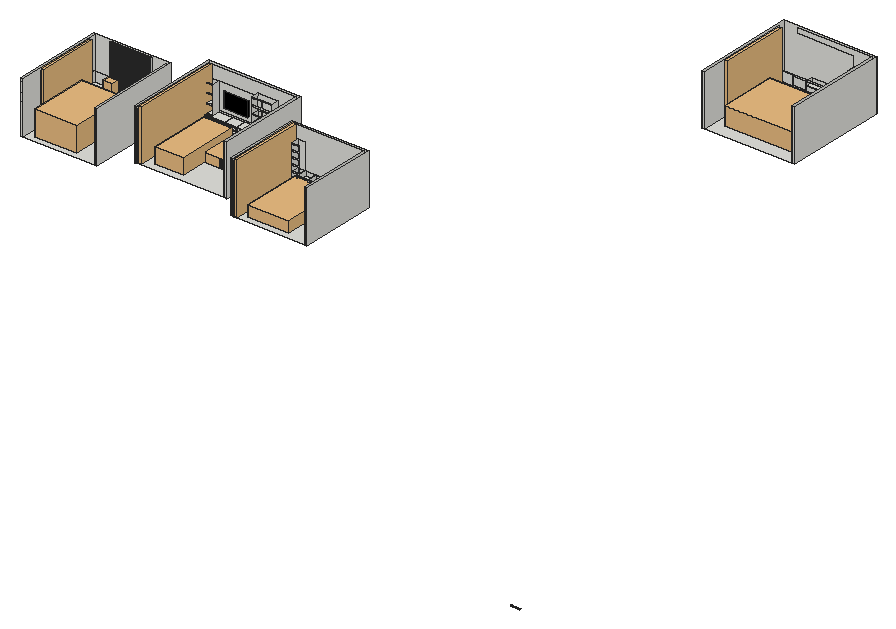
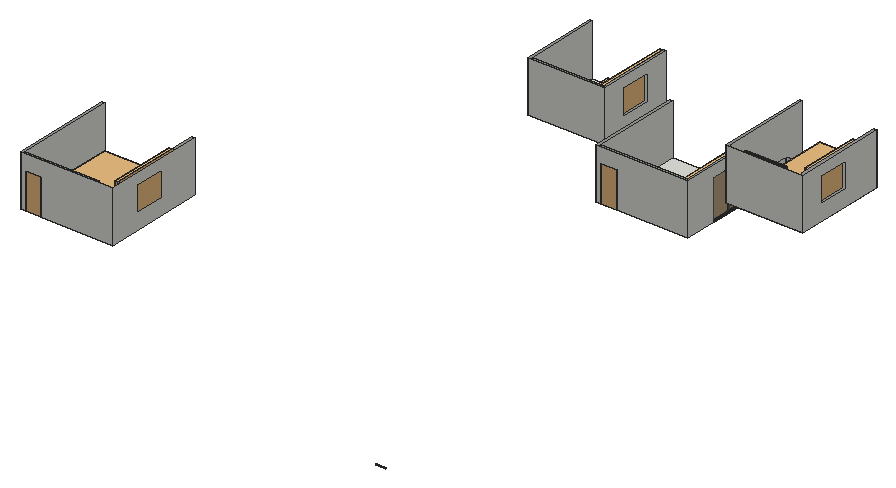
# SketchUp Ruby script. Lengths in inches.
U = 1.inch
M = Sketchup.active_model
def pt(a) = Geom::Point3d.new(a.map { |v| v * U })
def face(e, loops, mat)
  f = e.add_face(loops[0].map { |a| pt(a) })
  loops[1..].each { |l| e.add_face(l.map { |a| pt(a) }).erase! }
  f.material = f.back_material = mat if mat
  f
end
# faces: each face lists its corners as indices into pts; further lists are holes
def faces(e, pts, list, mat = nil) = list.each { |f| face(e, (f[0].is_a?(Array) ? f : [f]).map { |l| l.map { |i| pts[i] } }, mat) }
# xy, xz, yz: faces in a plane at the given z, y or x. An outline is a flat list of corners, or four numbers for a rectangle; further outlines are holes
def ring(l) = l.size == 4 ? [[l[0], l[1]], [l[2], l[1]], [l[2], l[3]], [l[0], l[3]]] : l.each_slice(2).to_a
def flat(e, list, mat, &to3) = list.each { |f| face(e, (f[0].is_a?(Array) ? f : [f]).map { |l| ring(l).map { |u, v| to3.(u, v) } }, mat) }
def xy(e, z, list, mat = nil) = flat(e, list, mat) { |x, y| [x, y, z] }
def xz(e, y, list, mat = nil) = flat(e, list, mat) { |x, z| [x, y, z] }
def yz(e, x, list, mat = nil) = flat(e, list, mat) { |y, z| [x, y, z] }
def lines(e, pts, list) = list.each { |a, b| e.add_line(pt(pts[a]), pt(pts[b])) }
# prism: a flat outline (further loops are holes) pulled along v
def prism(e, loops, v, mat = nil)
  f = face(e, loops, mat); d = Geom::Vector3d.new(v.map { |x| x * U })
  f.pushpull(f.normal.samedirection?(d) ? d.length : -d.length)
end
def box(e, o, s, mat = nil) = prism(e, [[o, [o[0] + s[0], o[1], o[2]], [o[0] + s[0], o[1] + s[1], o[2]], [o[0], o[1] + s[1], o[2]]]], [0, 0, s[2]], mat)
def at(x, y, z, deg = 0) = Geom::Transformation.translation(pt([x, y, z])) * Geom::Transformation.rotation(ORIGIN, Z_AXIS, deg.degrees)
def axes(o, x, y, z) = Geom::Transformation.new([*x, 0, *y, 0, *z, 0, *pt(o).to_a, 1])
def part(name) = M.definitions.add(name)
# library, detail: a bought-in or finely detailed component or shape, given as its bounding box
def library(name, o, s) = part(name).tap { |d| box(d.entities, o, s) }
def detail(e, o, s) = box(e.add_group.entities, o, s)
def put(e, d, t, mat = nil) = e.add_instance(d, t).tap { |i| i.material = mat if mat }
def group(e, t, mat = nil) = e.add_group.tap { |g| g.transformation = t; g.material = mat if mat }.entities
root = M.entities
M.materials.add("Chrome_Polished").color = [2, 2, 2]
M.materials.add("[0135_DarkGray]").color = [81, 81, 81]
M.materials.add("[0137_Black]").color = [0, 0, 0]
M.materials.add("[Translucent Glass Gray]").color = [128, 128, 128]
M.materials["[Translucent Glass Gray]"].alpha = 0.15
M.materials.add("blackened steel1").color = [30, 30, 30]
c1 = part("Horizontal batten")
box(c1.entities,[0,-1,0],[23,1,1])
c2 = library("Garniza_zaclona",[1.52,0,0],[127.96,8.15,78.72])
c3 = library("main+door",[0,-0.79,0],[47.24,7.88,82.68])
c4 = part("PENTEK_RP Fineline 50S_SlidingDoor_Glass")
box(c4.entities,[0,0,0],[46.58,0.16,94.39],"[Translucent Glass Gray]")
c5 = part("PENTEK_RP Fineline 50S_SlidingDoor_GlazingBead")
box(c5.entities,[0,0,0],[45.47,0.59,0.56],"[0135_DarkGray]")
c6 = part("PENTEK_RP Fineline 50S_SlidingDoor_GlazingBead_2")
box(c6.entities,[0,0,0],[0.56,0.59,94.39],"[0135_DarkGray]")
c7 = part("PENTEK_RP Fineline 50S_SlidingDoor_Leaf_E1")
xy(c7.entities,0,[[0,0,0.93,1.97],[0.93,1.57,1.49,1.97]],"[0135_DarkGray]")
xy(c7.entities,96.25,[[0,0,0.93,0,0.93,1.57,1.49,1.57,1.49,1.97,0,1.97]],"[0135_DarkGray]")
xz(c7.entities,0,[[0,0,0.93,96.25]],"[0135_DarkGray]")
xz(c7.entities,1.57,[[0.93,0,1.49,95.32],[0.93,95.32,1.49,96.25]],"[0135_DarkGray]")
xz(c7.entities,1.97,[[0,0,1.49,96.25]],"[0135_DarkGray]")
yz(c7.entities,0,[[0,0,1.97,96.25]],"[0135_DarkGray]")
yz(c7.entities,0.93,[[0,0,1.57,0.93],[0,0.93,1.57,95.32],[0,95.32,1.57,96.25]],"[0135_DarkGray]")
yz(c7.entities,1.49,[[1.57,0,1.97,95.32],[1.57,95.32,1.97,96.25]],"[0135_DarkGray]")
c8 = part("PENTEK_RP Fineline 50S_SlidingDoor_Leaf_E2")
xy(c8.entities,0,[[0,0,0,1.57,0.56,1.57,0.56,1.97,46.02,1.97,46.02,1.57,46.58,1.57,46.58,0]],"[0135_DarkGray]")
xy(c8.entities,0.93,[[0,0,46.58,1.57]],"[0135_DarkGray]")
xy(c8.entities,1.49,[[0.56,1.57,46.02,1.97]],"[0135_DarkGray]")
xz(c8.entities,0,[[0,0,46.58,0.93]],"[0135_DarkGray]")
xz(c8.entities,1.57,[[0,0,0.56,0.93],[46.02,0,46.58,0.93],[0.56,0.93,46.02,1.49]],"[0135_DarkGray]")
xz(c8.entities,1.97,[[0.56,0,46.02,1.49]],"[0135_DarkGray]")
yz(c8.entities,0,[[0,0,1.57,0.93]],"[0135_DarkGray]")
yz(c8.entities,0.56,[[1.57,0,1.97,0.93],[1.57,0.93,1.97,1.49]],"[0135_DarkGray]")
yz(c8.entities,46.02,[[1.57,0,1.97,0.93],[1.57,0.93,1.97,1.49]],"[0135_DarkGray]")
yz(c8.entities,46.58,[[0,0,1.57,0.93]],"[0135_DarkGray]")
c9 = part("PENTEK_RP Fineline 50S_SlidingDoor_Leaf2")
put(c9.entities,c4,at(1.49,1.42,0.93))
put(c9.entities,c5,at(1.49,0,94.77))
put(c9.entities,c6,at(46.96,0,0.93))
put(c9.entities,c4,at(1.49,0.59,0.93))
put(c9.entities,c6,at(0.93,0,0.93))
put(c9.entities,c7,at(0,0,0))
put(c9.entities,c7,axes([48.44,0,0],[-1,0,0],[0,1,0],[0,0,1]))
put(c9.entities,c5,at(1.49,0,0.93))
put(c9.entities,c8,axes([0.93,0,96.25],[1,0,0],[0,1,0],[0,0,-1]))
put(c9.entities,c8,at(0.93,0,0))
c10 = part("PENTEK_RP Fineline S_SlidingDoor_Leaf1")
put(c10.entities,c6,at(0.93,0,0.93))
put(c10.entities,c6,at(46.96,0,0.93))
put(c10.entities,c4,at(1.49,1.42,0.93))
put(c10.entities,c5,at(1.49,0,0.93))
put(c10.entities,c4,at(1.49,0.59,0.93))
put(c10.entities,c7,at(0,0,0))
put(c10.entities,c7,axes([48.44,0,0],[-1,0,0],[0,1,0],[0,0,1]))
put(c10.entities,c8,axes([0.93,0,96.25],[1,0,0],[0,1,0],[0,0,-1]))
put(c10.entities,c8,at(0.93,0,0))
put(c10.entities,c5,at(1.49,0,94.77))
c11 = part("PENTEK_RP Fineline 50S_Sliding_DoorCase_E1")
box(c11.entities,[0,0,0],[1.51,3.66,99.27],"[0135_DarkGray]")
c12 = part("PENTEK_RP Fineline 50S_SlidingDooe_Case_E2")
box(c12.entities,[0,0,0],[96.25,3.66,1.51],"[0135_DarkGray]")
c13 = part("pentek_RP Fineline 50S_SlidingDoor_Case")
put(c13.entities,c11,at(97.76,0,0))
put(c13.entities,c12,at(1.51,0,0))
put(c13.entities,c11,at(0,0,0))
put(c13.entities,c12,at(1.51,0,97.76))
c14 = library("2222",[-1.18,-2.36,0.79],[68.11,146.45,37.25])
c15 = library("Group\#8",[0,0,0],[54,72,22])
c16 = part("Vertical batten")
box(c16.entities,[0,-1,0],[1,1,17])
c17 = part("Vertical batten \#1")
box(c17.entities,[-1,0,0],[1,1,16])
c18 = library("Garniza_zaclona\#1",[1.52,0,0],[127.96,8.15,78.72])
c19 = library("Garniza_zaclona\#3",[1.52,0,0],[127.96,8.15,78.72])
c20 = library("Garniza_zaclona\#2",[1.52,0,0],[127.96,8.15,78.72])
c21 = library("04+Sofa+y+Mesas",[-94.93,-111.67,3.93],[153.81,110.61,64.28])
c22 = library("Sofa+Set+3+(1)",[-143.38,0,-0.17],[159.32,111.7,30.39])
c23 = library("sofa+(2)",[-100.93,-81.02,-0.06],[174.43,145.32,46.54])
c24 = library("SKT_Nearly Natural 5' Kentia Palm Silk Tree",[-23.18,-17.61,0],[47.48,43.95,59.125])
c25 = part("Vertical wall batten")
prism(c25.entities,[[[1,0,0],[0,0,0],[0,0,24],[0,0,25],[0,0,48.5],[0,0,49.5],[0,0,73],[0,0,74],[0,0,98],[1,0,98]]],[0,-1,0])
xy(root,-33.45,[[194.45,99.3,398.45,99.3,398.45,309.3,392.45,309.3,392.45,315.3,356.45,315.3,356.45,309.3,194.45,309.3,194.45,243.3,188.45,243.3,188.45,147.3,194.45,147.3]])
xy(root,-28.45,[[194.45,285.3,218.45,309.3],[218.45,285.3,308.45,309.3],[308.45,285.3,332.45,309.3],[332.45,285.3,356.45,309.3]])
xy(root,-27.45,[[218.45,285.3,248.45,285.48],[249.45,285.3,277.45,309.3],[278.45,285.3,332.45,285.48]])
xy(root,-27.25,[[218.65,285.3,248.25,285.48],[278.65,285.3,308.25,285.48],[308.65,285.3,332.25,285.48]])
xy(root,-19.95,[[249.45,285.3,277.45,309.3]])
xy(root,-18.95,[[249.45,285.3,277.45,309.3]])
xy(root,-11.65,[[218.65,285.3,248.25,285.48],[278.65,285.3,308.25,285.48],[308.65,285.3,332.25,285.48]])
xy(root,-11.45,[[218.45,285.3,248.45,285.48],[249.45,285.3,277.45,309.3],[278.45,285.3,332.45,285.48]])
xy(root,-10.45,[[194.45,285.3,356.45,285.3,356.45,291.3,308.45,291.3,308.45,309.3,218.45,309.3,218.45,291.3,194.45,291.3]])
xy(root,-9.45,[[195.45,291.3,217.45,307.3],[309.45,291.3,355.45,309.3]])
xy(root,-4.45,[[218.45,307.3,308.45,309.3]])
xy(root,0,[[0.24,0,6.24,0,6.24,210,174.24,210,174.24,0,180.24,0,180.24,216,0.24,216],[6.24,0,174.24,210],[492.34,7.4375,660.34,7.4375,660.34,181.4375,522.34,181.4375,522.34,163.4375,504.34,163.4375,504.34,181.4375,492.34,181.4375],[962.01,801.86,1166.01,801.86,1166.01,1035.86,1160.01,1035.86,1160.01,1041.86,1124.01,1041.86,1124.01,1035.86,962.01,1035.86]])
xy(root,1,[[505.34,163.4375,521.34,181.4375]])
xy(root,4,[[6.24,192,174.24,210]])
xy(root,5,[[7.24,192,173.24,192.18]])
xy(root,5.2,[[7.4375,192,42.04,192.18],[42.4375,192,90.04,192.18],[90.4375,192,138.04,192.18],[138.4375,192,173.04,192.18]])
xy(root,6,[[156.24,48,174.24,156],[522.34,157.62,547.84,181.4375],[547.84,157.62,573.34,181.4375],[573.34,157.62,598.84,181.4375],[598.84,157.62,624.34,181.4375],
  [962.01,1017.86,1124.01,1035.86]])
xy(root,6.2,[[522.54,157.4375,547.64,157.62],[548.04,157.4375,573.34,157.62],[573.34,157.4375,598.64,157.62],[599.04,157.4375,624.14,157.62]])
xy(root,7,[[963.01,1017.86,1123.01,1018.04]])
xy(root,7.05,[[309.45,291.3,331.95,309.3],[331.95,291.3,332.95,309.3],[332.95,291.3,355.45,309.3]])
xy(root,7.2,[[963.21,1017.86,994.8125,1018.04],[995.21,1017.86,1026.8125,1018.04],[1027.21,1017.86,1058.8125,1018.04],[1059.21,1017.86,1090.8125,1018.04],[1091.21,1017.86,1122.8125,1018.04]])
xy(root,8,[[156.24,85.33,174.24,118.67]])
xy(root,8.05,[[309.45,291.3,331.95,309.3],[332.95,291.3,355.45,309.3]])
xy(root,11.05,[[195.45,291.3,217.45,307.3]])
xy(root,12.05,[[195.45,291.3,217.45,307.3]])
xy(root,14.5,[[156.24,85.33,174.24,118.67]])
xy(root,15.17,[[505.34,163.4375,521.34,181.4375]])
xy(root,15.5,[[156.24,85.33,174.24,118.67]])
xy(root,16.17,[[505.34,163.4375,521.34,181.4375]])
xy(root,17.8,[[522.54,157.4375,547.64,157.62],[548.04,157.4375,598.64,157.62],[599.04,157.4375,624.14,157.62],[1027.21,1017.86,1058.8125,1018.04],[1059.21,1017.86,1090.8125,1018.04]])
xy(root,18,[[522.34,157.4375,624.34,157.62],[1027.01,1017.86,1091.01,1018.04]])
xy(root,19,[[523.34,157.4375,547.34,181.4375],[548.34,157.4375,598.34,181.4375],[599.34,157.4375,623.34,181.4375],[1028.01,1017.86,1090.01,1033.86]])
xy(root,20.8,[[7.4375,192,42.04,192.18],[42.4375,192,90.04,192.18],[90.4375,192,138.04,192.18],[138.4375,192,173.04,192.18]])
xy(root,21,[[7.24,192,173.24,192.18]])
xy(root,22,[[156.24,85.33,174.24,118.67],[6.24,192,174.24,210]])
xz(root,0,[[0.24,0,6.24,120],[174.24,0,180.24,120]])
xz(root,7.4375,[[486.34,0,492.34,120],[660.34,0,666.34,120]])
xz(root,48,[[156.24,6,174.24,24]])
xz(root,85.33,[[156.24,8,174.24,14.5],[156.24,15.5,174.24,22]])
xz(root,99.3,[[188.45,-34.45,194.45,-33.45,194.45,85.55,188.45,85.55],[404.45,-34.45,404.45,85.55,398.45,85.55,398.45,-33.45]])
xz(root,118.67,[[156.24,8,174.24,14.5],[156.24,15.5,174.24,22]])
xz(root,147.3,[[188.45,-33.45,194.45,61.55]])
xz(root,156,[[156.24,6,174.24,24]])
xz(root,157.4375,[[522.54,6.2,547.64,17.8],[548.04,6.2,598.64,17.8],[599.04,6.2,624.14,17.8],[[522.34,18,624.34,30],[523.34,19,623.34,29]],[547.34,19,548.34,29],
  [598.34,19,599.34,29]])
xz(root,157.62,[[[522.34,6,624.34,18],[548.04,6.2,598.64,17.8],[599.04,6.2,624.14,17.8],[522.54,6.2,547.64,17.8]]])
xz(root,163.4375,[[[504.34,0,522.34,90],[505.34,1,521.34,15.17],[505.34,74.83,521.34,89],[505.34,16.17,521.34,29.83],[505.34,45.5,521.34,59.17],[505.34,30.83,521.34,44.5],[505.34,60.17,521.34,73.83]]])
xz(root,181.4375,[[492.34,0,504.34,0,504.34,90,523.34,90,523.34,30,624.34,30,624.34,6,522.34,6,522.34,0,660.34,0,660.34,120,492.34,120],[505.34,1,521.34,15.17],[505.34,16.17,521.34,29.83],[523.34,19,547.34,29],[548.34,19,598.34,29],
  [599.34,19,623.34,29]])
xz(root,187.4375,[[486.34,0,666.34,120]])
xz(root,192,[[[6.24,4,174.24,22],[7.24,5,173.24,21]],[7.4375,5.2,42.04,20.8],[42.4375,5.2,90.04,20.8],[90.4375,5.2,138.04,20.8],[138.4375,5.2,173.04,20.8]])
xz(root,192.18,[[[7.24,5,173.24,21],[90.4375,5.2,138.04,20.8],[42.4375,5.2,90.04,20.8],[138.4375,5.2,173.04,20.8],[7.4375,5.2,42.04,20.8]]],"Chrome_Polished")
xz(root,210,[[6.24,0,174.24,4],[6.24,22,42.24,46],[42.24,22,43.24,120],[43.24,22,138.24,120],[138.24,22,174.24,46]])
xz(root,216,[[0.24,0,180.24,120]])
xz(root,243.3,[[188.45,-33.45,194.45,61.55]])
xz(root,285.3,[[[194.45,-28.45,218.45,-28.45,218.45,-27.45,195.45,-27.45,195.45,-11.45,248.45,-11.45,248.45,-27.45,218.45,-27.45,218.45,-28.45,332.45,-28.45,332.45,-27.45,278.45,-27.45,278.45,-11.45,355.45,-11.45,355.45,-27.45,332.45,-27.45,332.45,-28.45,356.45,-28.45,356.45,-10.45,194.45,-10.45],[249.45,-27.45,277.45,-11.45]],[195.45,-27.45,218.45,-12.45],[332.45,-27.45,355.45,-11.45],[218.65,-27.25,248.25,-11.65],[278.65,-27.25,308.25,-11.65],
  [308.65,-27.25,332.25,-11.65],[249.45,-19.95,277.45,-18.95]])
xz(root,285.48,[[[218.45,-27.45,248.45,-11.45],[218.65,-27.25,248.25,-11.65]],[[278.45,-27.45,332.45,-11.45],[278.65,-27.25,308.25,-11.65],[308.65,-27.25,332.25,-11.65]]])
xz(root,291.3,[[[194.45,-10.45,218.45,55.55],[195.45,12.05,217.45,33.05],[195.45,-9.45,217.45,11.05],[195.45,34.05,217.45,54.55]],[[308.45,-10.45,356.45,61.55],[309.45,8.05,309.45,25.05,331.95,25.05,331.95,8.05,332.95,8.05,332.95,25.05,355.45,25.05,355.45,8.05],[309.45,-9.45,355.45,7.05],[332.95,26.05,355.45,43.05],[309.45,26.05,331.95,43.05],[309.45,44.05,331.95,60.55],[332.95,44.05,355.45,60.55]]])
xz(root,307.3,[[195.45,-9.45,217.45,11.05],[218.45,-4.45,308.45,55.55],[195.45,12.05,217.45,33.05]])
xz(root,309.3,[[194.45,-33.45,356.45,-28.45],[392.45,-33.45,398.45,-33.45,398.45,85.55,195.45,85.55,195.45,55.55,308.45,55.55,308.45,61.55,356.45,61.55,356.45,49.55,392.45,49.55],[249.45,-27.45,277.45,-19.95],[249.45,-18.95,277.45,-11.45],[218.45,-10.45,308.45,-4.45],
  [309.45,-9.45,355.45,7.05],[309.45,8.05,331.95,25.05],[332.95,8.05,355.45,25.05]])
xz(root,315.3,[[188.45,-34.45,188.45,85.55,404.45,85.55,404.45,-34.45,392.45,-33.45,392.45,49.55,356.45,49.55,356.45,-33.45]])
xz(root,801.86,[[956.01,0,962.01,120],[1166.01,0,1172.01,120]])
xz(root,1017.86,[[[962.01,6,1124.01,30],[963.01,7,1123.01,29]],[963.21,7.2,994.8125,28.8],[995.21,7.2,1026.8125,28.8],[1027.21,7.2,1058.8125,17.8],[1059.21,7.2,1090.8125,17.8],
  [1091.21,7.2,1122.8125,28.8],[[1027.01,18,1091.01,29],[1028.01,19,1090.01,28]]])
xz(root,1018.04,[[[963.01,7,1123.01,7,1123.01,29,1091.01,29,1091.01,18,1027.01,18,1027.01,29,963.01,29],[963.21,7.2,994.8125,28.8],[995.21,7.2,1026.8125,28.8],[1091.21,7.2,1122.8125,28.8],[1059.21,7.2,1090.8125,17.8],[1027.21,7.2,1058.8125,17.8]]],"blackened steel1")
xz(root,1033.86,[[1028.01,19,1090.01,28]])
xz(root,1035.86,[[962.01,0,1124.01,6],[1160.01,0,1166.01,0,1166.01,120,992.01,120,992.01,108,1124.01,108,1124.01,84,1160.01,84]])
xz(root,1041.86,[[956.01,0,956.01,120,1172.01,120,1172.01,0,1160.01,0,1160.01,84,1124.01,84,1124.01,0]])
yz(root,0.24,[[[0,0,216,120],[90,36,162,96]]])
yz(root,6.24,[[[0,0,210,0,210,4,192,4,192,22,210,22,210,46,192,46,192,47,210,47,210,70.5,192,70.5,192,71.5,210,71.5,210,95,192,95,192,96,210,96,210,120,0,120],[90,36,162,96]]])
yz(root,7.24,[[192,5,192.18,21]])
yz(root,7.4375,[[192,5.2,192.18,20.8]])
yz(root,42.04,[[192,5.2,192.18,20.8]])
yz(root,42.4375,[[192,5.2,192.18,20.8]])
yz(root,90.04,[[192,5.2,192.18,20.8]])
yz(root,90.4375,[[192,5.2,192.18,20.8]])
yz(root,138.04,[[192,5.2,192.18,20.8]])
yz(root,138.4375,[[192,5.2,192.18,20.8]])
yz(root,156.24,[[[48,6,156,24],[49,7,155,23]],[49,7,84.33,23],[[84.33,7,119.67,23],[85.33,8,118.67,22]],[119.67,7,155,23],[85.33,14.5,118.67,15.5]])
yz(root,173.04,[[192,5.2,192.18,20.8]])
yz(root,173.24,[[192,5,192.18,21]])
yz(root,174.24,[[[0,0,0,120,210,120,210,96,192,96,192,95,210,95,210,71.5,192,71.5,192,70.5,210,70.5,210,47,192,47,192,46,210,46,210,22,192,22,192,4,210,4,210,0],[48,6,156,24]],[85.33,8,118.67,14.5],[85.33,15.5,118.67,22]])
yz(root,180.24,[[0,0,216,120]])
yz(root,188.45,[[[99.3,-34.45,315.3,85.55],[147.3,-33.45,243.3,61.55]]])
yz(root,194.45,[[99.3,-33.45,147.3,-33.45,147.3,61.55,243.3,61.55,243.3,-33.45,309.3,-33.45,309.3,-28.45,285.3,-28.45,285.3,-10.45,291.3,-10.45,291.3,55.55,309.3,55.55,309.3,85.55,99.3,85.55]])
yz(root,195.45,[[291.3,-9.45,307.3,11.05],[291.3,12.05,307.3,33.05]])
yz(root,217.45,[[291.3,-9.45,307.3,11.05],[291.3,12.05,307.3,33.05]])
yz(root,218.45,[[285.3,-27.45,285.48,-12.45],[285.3,-12.45,285.48,-11.45],[291.3,-10.45,309.3,-10.45,309.3,-4.45,307.3,-4.45,307.3,55.55,291.3,55.55]])
yz(root,218.65,[[285.3,-27.25,285.48,-12.45],[285.3,-12.45,285.48,-11.65]])
yz(root,248.25,[[285.3,-27.25,285.48,-11.65]])
yz(root,248.45,[[285.3,-27.45,285.48,-11.45]])
yz(root,249.45,[[285.3,-27.45,309.3,-19.95],[285.3,-18.95,309.3,-11.45]])
yz(root,277.45,[[285.3,-27.45,309.3,-19.95],[285.3,-18.95,309.3,-11.45]])
yz(root,278.45,[[285.3,-27.45,285.48,-11.45]])
yz(root,278.65,[[285.3,-27.25,285.48,-11.65]])
yz(root,308.25,[[285.3,-27.25,285.48,-11.65]])
yz(root,308.45,[[291.3,-10.45,291.3,61.55,309.3,61.55,309.3,55.55,307.3,55.55,307.3,-4.45,309.3,-4.45,309.3,-10.45]])
yz(root,308.65,[[285.3,-27.25,285.48,-11.65]])
yz(root,309.45,[[291.3,-9.45,309.3,7.05],[291.3,8.05,309.3,25.05]])
yz(root,331.95,[[291.3,8.05,309.3,25.05]])
yz(root,332.25,[[285.3,-27.25,285.48,-11.65]])
yz(root,332.45,[[285.3,-27.45,285.48,-11.45]])
yz(root,332.95,[[291.3,8.05,309.3,25.05]])
yz(root,355.45,[[291.3,-9.45,309.3,7.05],[291.3,8.05,309.3,25.05]])
yz(root,356.45,[[309.3,-33.45,315.3,-33.45,315.3,49.55,309.3,49.55,309.3,61.55,291.3,61.55,291.3,-10.45,285.3,-10.45,285.3,-28.45,309.3,-28.45]])
yz(root,392.45,[[309.3,-33.45,315.3,49.55]])
yz(root,398.45,[[99.3,-33.45,309.3,85.55]])
yz(root,404.45,[[99.3,-34.45,315.3,85.55]])
yz(root,486.34,[[[7.4375,0,187.4375,120],[61.4375,36,133.4375,96]]])
yz(root,492.34,[[[7.4375,0,181.4375,120],[61.4375,36,133.4375,96]]])
yz(root,504.34,[[163.4375,0,181.4375,90]])
yz(root,505.34,[[163.4375,1,181.4375,15.17],[163.4375,16.17,181.4375,29.83]])
yz(root,521.34,[[163.4375,1,181.4375,6],[163.4375,6,181.4375,15.17],[163.4375,16.17,181.4375,18],[163.4375,18,181.4375,29.83]])
yz(root,522.34,[[163.4375,0,181.4375,6],[157.62,6,163.4375,18],[157.4375,18,163.4375,30]])
yz(root,522.54,[[157.4375,6.2,157.62,17.8]])
yz(root,523.34,[[157.4375,19,181.4375,29]])
yz(root,547.34,[[157.4375,19,181.4375,29]])
yz(root,547.64,[[157.4375,6.2,157.62,17.8]])
yz(root,548.04,[[157.4375,6.2,157.62,17.8]])
yz(root,548.34,[[157.4375,19,181.4375,29]])
yz(root,598.34,[[157.4375,19,181.4375,29]])
yz(root,598.64,[[157.4375,6.2,157.62,17.8]])
yz(root,599.04,[[157.4375,6.2,157.62,17.8]])
yz(root,599.34,[[157.4375,19,181.4375,29]])
yz(root,623.34,[[157.4375,19,181.4375,29]])
yz(root,624.14,[[157.4375,6.2,157.62,17.8]])
yz(root,624.34,[[157.62,6,181.4375,6,181.4375,30,157.4375,30,157.4375,18,157.62,18]])
yz(root,660.34,[[7.4375,0,181.4375,120]])
yz(root,666.34,[[7.4375,0,187.4375,120]])
yz(root,956.01,[[[801.86,0,1041.86,120],[897.86,36,969.86,96]]])
yz(root,962.01,[[[801.86,0,1035.86,0,1035.86,6,1017.86,6,1017.86,120,801.86,120],[897.86,36,969.86,96]]])
yz(root,963.01,[[1017.86,7,1018.04,29]])
yz(root,963.21,[[1017.86,7.2,1018.04,28.8]])
yz(root,994.8125,[[1017.86,7.2,1018.04,28.8]])
yz(root,995.21,[[1017.86,7.2,1018.04,28.8]])
yz(root,1026.8125,[[1017.86,7.2,1018.04,28.8]])
yz(root,1027.01,[[1017.86,18,1018.04,29]])
yz(root,1027.21,[[1017.86,7.2,1018.04,17.8]])
yz(root,1028.01,[[1017.86,19,1033.86,28]])
yz(root,1058.8125,[[1017.86,7.2,1018.04,17.8]])
yz(root,1059.21,[[1017.86,7.2,1018.04,17.8]])
yz(root,1090.01,[[1017.86,19,1033.86,28]])
yz(root,1090.8125,[[1017.86,7.2,1018.04,17.8]])
yz(root,1091.01,[[1017.86,18,1018.04,29]])
yz(root,1091.21,[[1017.86,7.2,1018.04,18],[1017.86,18,1018.04,28.8]])
yz(root,1122.8125,[[1017.86,7.2,1018.04,28.8]])
yz(root,1123.01,[[1017.86,7,1018.04,29]])
yz(root,1124.01,[[1035.86,0,1041.86,0,1041.86,84,1018.86,84,1018.86,78,1033.86,78,1033.86,30,1017.86,30,1017.86,6,1035.86,6]])
yz(root,1160.01,[[1035.86,0,1041.86,84]])
yz(root,1166.01,[[801.86,0,1035.86,120]])
yz(root,1172.01,[[801.86,0,1041.86,120]])
put(root,c1,at(921,285.3,-788))
put(root,c2,axes([202.6,99.3,-33.45],[0,1.62,0],[-1,0,0],[0,0,1.51175]))
put(root,c3,axes([356.45,312.3,-33.45],[0.762,0,0],[0,0.4697,0],[0,0,1.0039]))
g1 = group(root,at(192.57,147.3,-33.45))
put(g1,c9,axes([-1.26,47.69,1.44],[0,0.96704,0],[-0.64,0,0],[0,0,0.95696]))
put(g1,c10,axes([0,1.46,1.44],[0,0.96704,0],[-0.64,0,0],[0,0,0.95696]))
put(g1,c13,axes([-0.25,0,0],[0,0.96704,0],[-0.64,0,0],[0,0,0.95696]))
put(root,c14,axes([223.83,118.61,-33.57],[0.9758,0,0],[0,0.9758,0],[0,0,0.9758]))
put(root,c15,axes([342.36,177.99,-10.45],[-1,0,0],[0,1,0],[0,0,-1.0093]))
put(root,c16,at(324.36,178.99,-31.65))
put(root,c16,at(325.5625,178.99,-31.65))
put(root,c16,at(326.76,178.99,-31.65))
put(root,c16,at(327.96,178.99,-31.65))
put(root,c16,at(329.16,178.99,-31.65))
put(root,c16,at(330.36,178.99,-31.65))
put(root,c16,at(331.5625,178.99,-31.65))
put(root,c16,at(332.76,178.99,-31.65))
put(root,c16,at(333.96,178.99,-31.65))
put(root,c16,at(335.16,178.99,-31.65))
put(root,c16,at(336.36,178.99,-31.65))
put(root,c17,at(289.36,232.1875,-30.65))
put(root,c17,at(289.36,240.59,-30.65))
put(root,c17,at(289.36,239.39,-30.65))
put(root,c17,at(289.36,238.1875,-30.65))
put(root,c17,at(289.36,236.99,-30.65))
put(root,c17,at(289.36,235.79,-30.65))
put(root,c17,at(289.36,234.59,-30.65))
put(root,c17,at(289.36,233.39,-30.65))
put(root,c17,at(289.36,241.79,-30.65))
put(root,c17,at(289.36,242.99,-30.65))
put(root,c1,at(195.45,285.3,-28.05))
put(root,c1,at(332.45,285.3,-28.05))
put(root,c1,at(195.45,285.3,-26.85))
put(root,c1,at(332.45,285.3,-26.85))
put(root,c1,at(195.45,285.3,-25.65))
put(root,c1,at(332.45,285.3,-25.65))
put(root,c1,at(195.45,285.3,-24.45))
put(root,c1,at(332.45,285.3,-24.45))
put(root,c1,at(195.45,285.3,-23.25))
put(root,c1,at(332.45,285.3,-23.25))
put(root,c1,at(195.45,285.3,-22.05))
put(root,c1,at(332.45,285.3,-22.05))
put(root,c1,at(195.45,285.3,-20.85))
put(root,c1,at(332.45,285.3,-20.85))
put(root,c1,at(195.45,285.3,-19.65))
put(root,c1,at(332.45,285.3,-19.65))
put(root,c1,at(195.45,285.3,-18.45))
put(root,c1,at(332.45,285.3,-18.45))
put(root,c1,at(195.45,285.3,-17.25))
put(root,c1,at(332.45,285.3,-17.25))
put(root,c1,at(195.45,285.3,-16.05))
put(root,c1,at(332.45,285.3,-16.05))
put(root,c1,at(195.45,285.3,-14.85))
put(root,c1,at(332.45,285.3,-14.85))
put(root,c1,at(195.45,285.3,-13.65))
put(root,c1,at(332.45,285.3,-13.65))
put(root,c1,at(195.45,285.3,-12.45))
put(root,c1,at(332.45,285.3,-12.45))
put(root,c18,axes([500.49,7.4375,-2.01],[0,1.36,0],[-1,0,0],[0,0,1.55]))
put(root,c19,axes([970.16,857.02,0],[0,1.23451,0],[-1,0,0],[0,0,1.52445]))
put(root,c20,axes([14.39,50.59,0],[0,1.1,0],[-1,0,0],[0,0,1.52445]))
put(root,c3,axes([1124.01,1038.86,0],[0.762,0,0],[0,0.21899,0],[0,0,1.016]))
put(root,c21,axes([22.18,98.11,-3.54],[0,0.9,0],[-0.9,0,0],[0,0,0.9]))
put(root,c22,axes([611.13,146.28,0.14],[0,0.86,0],[-0.86,0,0],[0,0,0.86]))
put(root,c23,axes([1049.55,891.99,0.05],[-0.9085,0,0],[0,-0.9085,0],[0,0,0.9085]))
g2 = group(root,at(290.87,303.3,6.21),"[0137_Black]")
xy(g2,0,[[-57.42,0,0,2]])
xy(g2,13.93,[[-35.09,2,-23.29,4]])
xy(g2,20.17,[[-35.09,2,-23.29,4]])
xy(g2,35.38,[[-57.42,0,0,2]])
xz(g2,0,[[-57.42,0,0,35.38]])
xz(g2,2,[[[-57.42,0,0,35.38],[-35.09,13.93,-23.29,20.17]]])
xz(g2,4,[[-35.09,13.93,-23.29,20.17]])
yz(g2,-57.42,[[0,0,2,35.38]])
yz(g2,-35.09,[[2,13.93,4,20.17]])
yz(g2,-23.29,[[2,13.93,4,20.17]])
yz(g2,0,[[0,0,2,35.38]])
put(root,c24,axes([52.12,197.47,21.625],[0.4347,0,0],[0,0.4347,0],[0,0,0.4347]))
put(root,c25,at(42.24,210,22))
put(root,c25,at(43.4375,210,22))
put(root,c25,at(44.64,210,22))
put(root,c25,at(45.84,210,22))
put(root,c25,at(47.04,210,22))
put(root,c25,at(48.24,210,22))
put(root,c25,at(49.4375,210,22))
put(root,c25,at(50.64,210,22))
put(root,c25,at(51.84,210,22))
put(root,c25,at(53.04,210,22))
put(root,c25,at(54.24,210,22))
put(root,c25,at(55.4375,210,22))
put(root,c25,at(56.64,210,22))
put(root,c25,at(57.84,210,22))
put(root,c25,at(59.04,210,22))
put(root,c25,at(60.24,210,22))
put(root,c25,at(61.4375,210,22))
put(root,c25,at(62.64,210,22))
put(root,c25,at(63.84,210,22))
put(root,c25,at(65.04,210,22))
put(root,c25,at(66.24,210,22))
put(root,c25,at(67.4375,210,22))
put(root,c25,at(68.64,210,22))
put(root,c25,at(69.84,210,22))
put(root,c25,at(71.04,210,22))
put(root,c25,at(72.24,210,22))
put(root,c25,at(73.4375,210,22))
put(root,c25,at(74.64,210,22))
put(root,c25,at(75.84,210,22))
put(root,c25,at(77.04,210,22))
put(root,c25,at(78.24,210,22))
put(root,c25,at(79.4375,210,22))
put(root,c25,at(80.64,210,22))
put(root,c25,at(81.84,210,22))
put(root,c25,at(83.04,210,22))
put(root,c25,at(84.24,210,22))
put(root,c25,at(85.4375,210,22))
put(root,c25,at(86.64,210,22))
put(root,c25,at(87.84,210,22))
put(root,c25,at(89.04,210,22))
put(root,c25,at(90.24,210,22))
put(root,c25,at(91.4375,210,22))
put(root,c25,at(92.64,210,22))
put(root,c25,at(93.84,210,22))
put(root,c25,at(95.04,210,22))
put(root,c25,at(96.24,210,22))
put(root,c25,at(97.4375,210,22))
put(root,c25,at(98.64,210,22))
put(root,c25,at(99.84,210,22))
put(root,c25,at(101.04,210,22))
put(root,c25,at(102.24,210,22))
put(root,c25,at(103.4375,210,22))
put(root,c25,at(104.64,210,22))
put(root,c25,at(105.84,210,22))
put(root,c25,at(107.04,210,22))
put(root,c25,at(108.24,210,22))
put(root,c25,at(109.4375,210,22))
put(root,c25,at(110.64,210,22))
put(root,c25,at(111.84,210,22))
put(root,c25,at(113.04,210,22))
put(root,c25,at(114.24,210,22))
put(root,c25,at(115.4375,210,22))
put(root,c25,at(116.64,210,22))
put(root,c25,at(117.84,210,22))
put(root,c25,at(119.04,210,22))
put(root,c25,at(120.24,210,22))
put(root,c25,at(121.4375,210,22))
put(root,c25,at(122.64,210,22))
put(root,c25,at(123.84,210,22))
put(root,c25,at(125.04,210,22))
put(root,c25,at(126.24,210,22))
put(root,c25,at(127.4375,210,22))
put(root,c25,at(128.64,210,22))
put(root,c25,at(129.84,210,22))
put(root,c25,at(131.04,210,22))
put(root,c25,at(132.24,210,22))
put(root,c25,at(133.4375,210,22))
put(root,c25,at(134.64,210,22))
put(root,c25,at(135.84,210,22))
put(root,c25,at(137.04,210,22))
put(root,c25,at(138.24,210,22))
